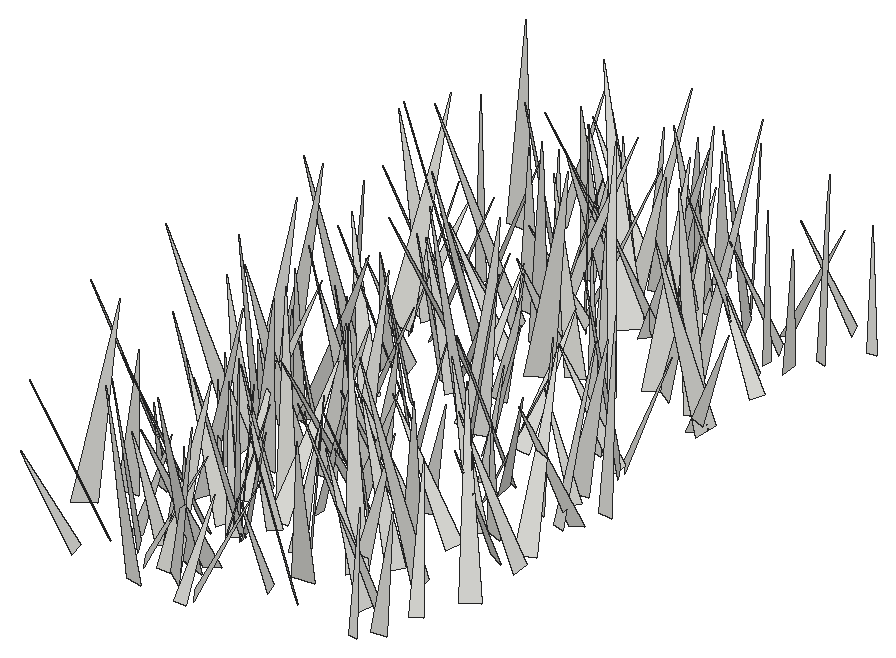
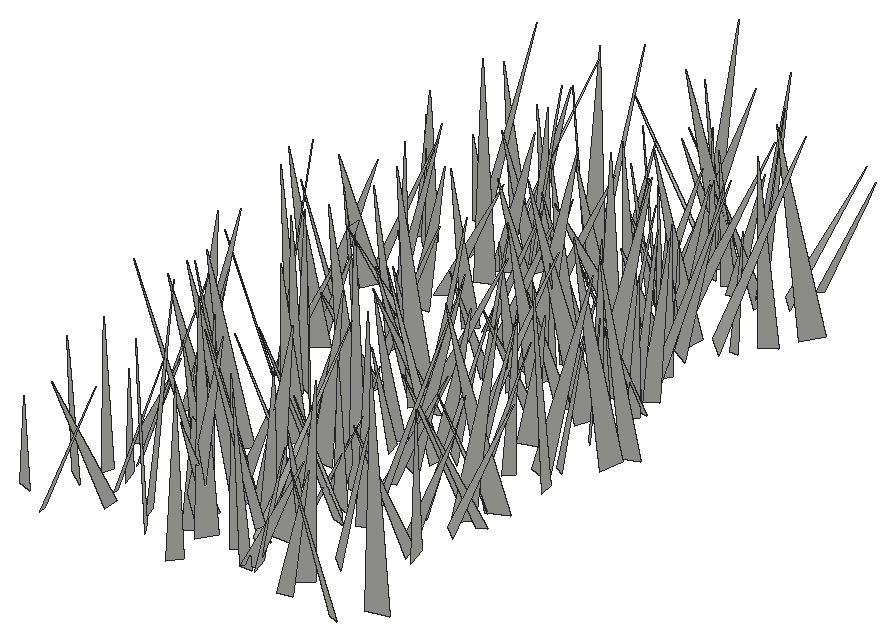
# SketchUp Ruby script. Lengths in inches.
U = 1.inch
M = Sketchup.active_model
def pt(a) = Geom::Point3d.new(a.map { |v| v * U })
def face(e, loops, mat)
  f = e.add_face(loops[0].map { |a| pt(a) })
  loops[1..].each { |l| e.add_face(l.map { |a| pt(a) }).erase! }
  f.material = f.back_material = mat if mat
  f
end
# faces: each face lists its corners as indices into pts; further lists are holes
def faces(e, pts, list, mat = nil) = list.each { |f| face(e, (f[0].is_a?(Array) ? f : [f]).map { |l| l.map { |i| pts[i] } }, mat) }
# xy, xz, yz: faces in a plane at the given z, y or x. An outline is a flat list of corners, or four numbers for a rectangle; further outlines are holes
def ring(l) = l.size == 4 ? [[l[0], l[1]], [l[2], l[1]], [l[2], l[3]], [l[0], l[3]]] : l.each_slice(2).to_a
def flat(e, list, mat, &to3) = list.each { |f| face(e, (f[0].is_a?(Array) ? f : [f]).map { |l| ring(l).map { |u, v| to3.(u, v) } }, mat) }
def xy(e, z, list, mat = nil) = flat(e, list, mat) { |x, y| [x, y, z] }
def xz(e, y, list, mat = nil) = flat(e, list, mat) { |x, z| [x, y, z] }
def yz(e, x, list, mat = nil) = flat(e, list, mat) { |y, z| [x, y, z] }
def lines(e, pts, list) = list.each { |a, b| e.add_line(pt(pts[a]), pt(pts[b])) }
# prism: a flat outline (further loops are holes) pulled along v
def prism(e, loops, v, mat = nil)
  f = face(e, loops, mat); d = Geom::Vector3d.new(v.map { |x| x * U })
  f.pushpull(f.normal.samedirection?(d) ? d.length : -d.length)
end
def box(e, o, s, mat = nil) = prism(e, [[o, [o[0] + s[0], o[1], o[2]], [o[0] + s[0], o[1] + s[1], o[2]], [o[0], o[1] + s[1], o[2]]]], [0, 0, s[2]], mat)
def at(x, y, z, deg = 0) = Geom::Transformation.translation(pt([x, y, z])) * Geom::Transformation.rotation(ORIGIN, Z_AXIS, deg.degrees)
def axes(o, x, y, z) = Geom::Transformation.new([*x, 0, *y, 0, *z, 0, *pt(o).to_a, 1])
def part(name) = M.definitions.add(name)
# library, detail: a bought-in or finely detailed component or shape, given as its bounding box
def library(name, o, s) = part(name).tap { |d| box(d.entities, o, s) }
def detail(e, o, s) = box(e.add_group.entities, o, s)
def put(e, d, t, mat = nil) = e.add_instance(d, t).tap { |i| i.material = mat if mat }
def group(e, t, mat = nil) = e.add_group.tap { |g| g.transformation = t; g.material = mat if mat }.entities
root = M.entities
c1 = part("fur_instance\#9")
p = [[0.8125,0,1.79],[0.67,-0.02,1.48],[0,-0.11,0],[0,0.11,0]]
faces(c1.entities,p,[[0,1,2,3]])
put(root,c1,axes([480.35,103.58,-21.66],[1.05516,-7.50337,2.43147],[-7.87164,-0.84629,0.8044],[0.49989,2.51181,7.53438]))
put(root,c1,axes([480.21,79.61,-21.66],[0.14436,6.2225,2.72909],[6.68972,0.34776,-1.14678],[1.18962,-2.71069,6.11762]))
put(root,c1,axes([483.13,93.17,-21.66],[-3.10953,-4.00727,0.37973],[-3.98696,3.00024,-0.98706],[-0.55366,0.90108,4.97525]))
put(root,c1,axes([480.6,81.01,-21.66],[7.15421,-1.9799,2.12173],[-2.22149,-7.36827,0.61487],[-1.86728,1.18029,7.39761]))
put(root,c1,axes([483.24,84.46,-21.66],[-1.73003,-6.76572,2.01517],[-7.01807,1.42401,-1.24409],[-0.76325,2.2419,6.8717]))
put(root,c1,axes([480.98,61.46,-21.66],[5.12672,-4.5376,2.59386],[-5.0883,-5.16347,1.02416],[-1.19461,2.5199,6.76936]))
put(root,c1,axes([482.8,96.8125,-21.66],[-5.66532,-0.50223,1.85308],[-0.88322,5.80808,-1.12609],[1.70472,1.34012,5.57494]))
put(root,c1,axes([484.51,72.17,-21.66],[-7.8071,-1.03462,1.04066],[-0.93299,7.84786,0.80297],[1.13267,-0.66693,7.83431]))
put(root,c1,axes([483.31,91.69,-21.66],[-5.98098,3.27291,2.42019],[3.72115,6.13978,0.89298],[1.64993,-1.98304,6.75918]))
put(root,c1,axes([484.76,59.01,-21.66],[-3.76268,-4.24685,0.11424],[-4.17448,3.66755,-1.15295],[-0.78896,0.84846,5.55555]))
put(root,c1,axes([482.75,83.29,-21.66],[-2.78076,-3.999,1.01738],[-3.97731,2.92434,0.62365],[1.09912,0.46468,4.83071]))
put(root,c1,axes([484.81,65.8,-21.66],[-4.99858,-6.00178,0.67378],[-6.03784,4.94565,-0.739],[-0.1407,0.9901,7.77567]))
put(root,c1,axes([481.91,85.54,-21.66],[6.17707,1.48648,1.9777],[1.80034,-6.34915,-0.85095],[-1.69697,-1.32504,6.29616]))
put(root,c1,axes([482.12,79.45,-21.66],[3.64013,-0.49009,0.65042],[-0.33955,-3.62113,-0.82821],[-0.74023,-0.74902,3.57838]))
put(root,c1,axes([482.29,89.69,-21.66],[-1.03239,7.59334,1.92082],[7.72051,1.31303,-1.04105],[1.31985,-1.74108,7.59215]))
put(root,c1,axes([484.16,56.68,-21.66],[-3.93279,-0.23592,0.50656],[-0.05149,3.7386,1.34138],[0.55643,-1.32147,3.70448]))
put(root,c1,axes([481.97,91.59,-21.66],[0.26684,4.21608,0.5662],[4.07293,-0.08948,-1.25314],[1.22767,-0.6195,4.03438]))
put(root,c1,axes([482.01,105.68,-21.66],[2.56604,4.25646,1.10853],[4.39439,-2.42581,-0.85772],[0.18887,-1.38883,4.89555]))
put(root,c1,axes([483.74,73.5,-21.66],[3.52477,-3.78027,2.43443],[-3.94318,-4.08529,-0.63451],[-2.1606,1.28874,5.1295]))
put(root,c1,axes([484.54,73.62,-21.66],[-3.5063,-5.04513,2.56803],[-5.65565,3.25438,-1.32851],[0.24851,2.88062,5.99854]))
put(root,c1,axes([482.27,63.98,-21.66],[2.19919,-5.46865,1.19281],[-5.58851,-2.07385,0.79564],[0.31218,1.39943,5.84033]))
put(root,c1,axes([483.25,89.46,-21.66],[3.76197,3.17485,0.58422],[2.97684,-3.75885,1.25811],[-1.24876,0.60394,4.75913]))
put(root,c1,axes([483.43,79.5625,-21.66],[-2.68709,-2.60275,1.28992],[-2.48203,2.97011,0.82256],[1.50922,0.25052,3.6494]))
put(root,c1,axes([484.4,95.37,-21.66],[1.61464,-3.26071,0.69447],[-2.99454,-1.75765,-1.29032],[-1.46534,-0.00102,3.40211]))
put(root,c1,axes([485.8,92.11,-21.66],[-5.67662,-5.13617,1.32256],[-5.29359,5.60645,-0.94818],[0.32758,1.59402,7.59639]))
put(root,c1,axes([483.55,65.67,-21.66],[-0.85908,-3.57953,0.71794],[-3.54097,0.99653,0.73143],[0.88884,0.51028,3.60778]))
put(root,c1,axes([483.27,75.56,-21.66],[4.01305,-1.4697,0.35123],[-1.33059,-3.90931,-1.15533],[-0.71618,-0.97223,4.11458]))
put(root,c1,axes([485.89,100.32,-21.66],[-3.65286,-4.07637,1.60167],[-4.37583,3.48496,-1.11027],[0.18514,1.94004,5.3598]))
put(root,c1,axes([483.44,96.63,-21.66],[4.63443,1.21877,0.59299],[1.09033,-4.6073,0.94811],[-0.80513,0.77609,4.69728]))
put(root,c1,axes([486.17,82.04,-21.66],[-2.8304,4.89567,0.80261],[4.94903,2.72215,0.8485],[-0.34477,-1.11592,5.59096]))
put(root,c1,axes([485.76,68.05,-21.66],[-2.42816,-5.42807,1.43938],[-5.61543,2.33238,-0.67728],[-0.05217,1.5899,5.90772]))
put(root,c1,axes([483.19,74.81,-21.66],[2.79379,4.96818,0.70977],[4.95175,-2.59669,-1.31495],[0.8165,-1.25148,5.54607]))
put(root,c1,axes([484.66,77.3,-21.66],[-1.17903,-5.46423,1.73554],[-5.62366,1.44698,0.7353],[1.11548,1.51937,5.54141]))
put(root,c1,axes([486.03,86.25,-21.66],[-4.24869,-0.73201,1.00331],[-0.4187,4.21079,1.29914],[1.16925,-1.15205,4.11089]))
put(root,c1,axes([484.76,70.5,-21.66],[4.55576,-0.64185,1.19418],[-0.37344,-4.61891,-1.05794],[-1.3033,-0.92017,4.47746]))
put(root,c1,axes([484.73,85.62,-21.66],[4.79188,-1.27621,1.00499],[-1.01396,-4.79557,-1.25507],[-1.26909,-0.98723,4.79746]))
put(root,c1,axes([486.05,105.22,-21.66],[1.60844,-3.68609,1.55705],[-3.78668,-1.94455,-0.69177],[-1.29334,1.10916,3.96179]))
put(root,c1,axes([484.82,89.73,-21.66],[4.77629,1.47467,0.59608],[1.29577,-4.70156,1.24867],[-0.92247,1.03128,4.84029]))
put(root,c1,axes([486.55,74.48,-21.66],[1.44091,-6.85532,1.40735],[-6.89305,-1.6385,-0.92385],[-1.20912,1.1714,6.94393]))
put(root,c1,axes([488.1,93.9,-21.66],[-7.76303,-2.55675,1.09489],[-2.43873,7.81802,0.96517],[1.33728,-0.58482,8.11604]))
put(root,c1,axes([486.87,59.31,-21.66],[-4.89402,-3.33819,1.83703],[-3.30827,5.20635,0.64726],[1.89038,0.46913,5.88863]))
put(root,c1,axes([488.79,63.35,-21.66],[-3.68425,-5.36529,0.32526],[-5.32374,3.58793,-1.11818],[-0.74155,0.8979,6.41168]))
put(root,c1,axes([485.87,60.32,-21.66],[3.36091,-1.13304,0.9234],[-1.35023,-3.29337,0.87337],[-0.55977,1.1411,3.43755]))
put(root,c1,axes([486.125,103.26,-21.66],[4.8862,-3.80667,1.31151],[-3.74132,-5.05482,-0.73291],[-1.48774,0.20937,6.1505]))
put(root,c1,axes([487.35,66.4,-21.66],[-3.69275,-0.52533,1.17947],[-0.76187,3.77166,-0.70545],[1.04243,0.89562,3.66261]))
put(root,c1,axes([486.04,66.42,-21.66],[6.43486,-0.85229,1.84553],[-1.08084,-6.62327,0.70985],[-1.72168,0.97247,6.45212]))
put(root,c1,axes([488.4375,86.17,-21.66],[-2.6227,-3.62693,1.52989],[-3.9333,2.34177,-1.19122],[-0.15598,1.93268,4.31442]))
put(root,c1,axes([487.82,60.39,-21.66],[1.8485,-3.49978,1.33816],[-3.45042,-2.17169,-0.91344],[-1.46071,0.70098,3.8511]))
put(root,c1,axes([488.59,83,-21.66],[-3.38469,-3.26483,1.22467],[-3.48648,3.19729,-1.11215],[0.05857,1.65326,4.56929]))
put(root,c1,axes([489.88,103.8125,-21.66],[-3.98181,3.20015,0.16473],[3.12043,3.81261,1.36007],[-0.7287,-1.16015,4.92402]))
put(root,c1,axes([489.1,64.66,-21.66],[-4.79619,2.23097,0.90337],[2.34699,4.78153,0.65218],[0.53379,-0.97799,5.24932]))
put(root,c1,axes([489.59,90.88,-21.66],[-4.14397,2.00475,0.46664],[2.04964,3.92263,1.34951],[-0.1891,-1.41534,4.40117]))
put(root,c1,axes([488.96,74.16,-21.66],[0.98464,3.25356,1.70885],[3.23357,-1.6077,1.19779],[-1.74639,-1.14237,3.18127]))
put(root,c1,axes([490.18,81.1,-21.66],[-4.77204,-4.71706,0.72174],[-4.75307,4.60775,-1.31181],[-0.42413,1.43592,6.58044]))
put(root,c1,axes([489.4,103.45,-21.66],[-5.02924,-0.94611,0.83871],[-1.10156,4.96734,-1.00192],[0.62059,1.14984,5.01842]))
put(root,c1,axes([485.13,77.6,-21.66],[6.73019,-3.63445,0.24466],[-3.63894,-6.68481,0.79754],[0.16506,0.81773,7.60715]))
put(root,c1,axes([488.13,67.47,-21.66],[-2.89622,3.26829,0.45856],[3.08153,2.89643,-1.18106],[1.18158,0.4572,4.20415]))
put(root,c1,axes([486.59,71.41,-21.66],[1.17018,-6.95871,1.51726],[-7.0392,-0.89595,1.31981],[1.08411,1.69372,6.93189]))
put(root,c1,axes([487.09,77.39,-21.66],[3.48145,-1.92251,0.90917],[-2.10367,-3.36896,0.93158],[-0.31179,1.26381,3.86636]))
put(root,c1,axes([487.35,95.8,-21.66],[0.93072,-6.54849,1.55591],[-6.7031,-0.75944,0.81335],[0.60996,1.64631,6.5641]))
put(root,c1,axes([489.62,88.78,-21.66],[-2.51805,-6.35566,1.6356],[-6.55451,2.34778,-0.96776],[-0.32873,1.87181,6.76746]))
put(root,c1,axes([488.78,69.36,-21.66],[-4.40075,-1.21691,1.44212],[-0.98766,4.60363,0.87078],[1.60783,-0.50284,4.4821]))
put(root,c1,axes([489.28,55.73,-21.66],[1.25077,5.74635,3.18749],[6.40163,-1.79789,0.7292],[-1.48314,-2.91412,5.83551]))
put(root,c1,axes([487.46,101.11,-21.66],[2.40925,-3.29701,1.00546],[-3.44676,-2.29271,0.74099],[0.03277,1.24857,4.01568]))
put(root,c1,axes([487.72,79.45,-21.66],[4.13014,0.16234,0.60229],[0.00137,-4.03539,1.07832],[-0.62379,1.06603,3.99019]))
put(root,c1,axes([489.79,85.53,-21.66],[-3.61147,3.35043,1.62323],[3.67501,3.56996,0.80783],[0.59541,-1.71259,4.85958]))
put(root,c1,axes([489.76,75.13,-21.66],[1.9045,4.44389,1.45881],[4.34306,-2.26488,1.22946],[-1.73613,-0.79091,4.67587]))
put(root,c1,axes([490.43,63.66,-21.66],[-4.5545,1.12209,0.15618],[1.0267,4.36161,-1.39615],[0.47894,1.3207,4.4781]))
put(root,c1,axes([490.03,64.59,-21.66],[-4.76219,-1.42096,1.84075],[-1.91994,4.76946,-1.2853],[1.31199,1.82182,4.80058]))
put(root,c1,axes([490.82,64.08,-21.66],[-2.4507,-4.58404,1.24543],[-4.71435,2.17524,-1.27033],[-0.58261,1.68089,5.0404]))
put(root,c1,axes([490,94.97,-21.66],[1.00537,5.49165,1.69021],[5.63183,-1.28199,0.81538],[-1.13911,-1.49133,5.52306]))
put(root,c1,axes([491.95,85.92,-21.66],[-3.14306,-6.22127,0.26286],[-6.12359,3.03481,-1.39417],[-1.12913,0.859,6.8293]))
put(root,c1,axes([490.93,96.86,-21.66],[-3.84083,-1.16764,0.10273],[-1.10793,3.73134,0.98769],[0.38264,-0.91633,3.89099]))
put(root,c1,axes([491.39,101.33,-21.66],[-5.30348,-5.59312,0.1785],[-5.55783,5.29332,0.73008],[0.65218,-0.37354,7.67313]))
put(root,c1,axes([489.15,95.95,-21.66],[3.76049,3.04894,0.61025],[2.98388,-3.80785,0.6375],[-0.87456,0.11813,4.79905]))
put(root,c1,axes([490.78,68.4,-21.66],[-0.82841,6.75025,1.93378],[7.00258,0.65031,0.72978],[-0.51887,-2.00072,6.76162]))
put(root,c1,axes([488.95,59.54,-21.66],[1.24719,-3.91493,0.4967],[-3.8954,-1.13791,0.81231],[0.63182,0.71228,4.02769]))
put(root,c1,axes([490.55,100.1,-21.66],[1.73584,-5.70606,0.92261],[-5.63591,-1.88469,-1.0526],[-1.28332,0.55882,5.87063]))
put(root,c1,axes([489.92,63.84,-21.66],[3.50829,2.33455,0.59392],[2.17247,-3.51961,1.00185],[-1.04078,0.52272,4.09323]))
put(root,c1,axes([490.28,75.94,-21.66],[-4.55508,3.55475,2.05706],[3.40532,4.98624,-1.07596],[2.29598,-0.34303,5.67691]))
put(root,c1,axes([488.2,58.13,-21.66],[4.34126,2.62004,0.01209],[2.52851,-4.18338,-1.34808],[0.68659,-1.1602,4.88813]))
put(root,c1,axes([489.87,104.11,-21.66],[-1.04898,-5.12431,2.12616],[-5.35306,1.50327,0.98203],[1.45734,1.83333,5.13756]))
put(root,c1,axes([490.1875,59.51,-21.66],[-1.33091,-4.34516,1.37723],[-4.35803,1.6335,0.94222],[1.33595,0.99989,4.44566]))
put(root,c1,axes([493.18,97.96,-21.66],[-5.00695,6.61488,0.9269],[6.67749,4.92855,0.89773],[-0.16413,-1.27989,8.24744]))
put(root,c1,axes([491.8125,60.0625,-21.66],[0.91658,-6.09487,0.23316],[-5.96683,-0.94489,-1.24341],[-1.26442,0.04079,6.03668]))
put(root,c1,axes([491.44,75.21,-21.66],[2.47706,-6.70826,1.39737],[-6.69174,-2.68793,-1.04158],[-1.47445,0.92925,7.07472]))
put(root,c1,axes([489.02,96.39,-21.66],[3.55811,5.92159,0.8478],[5.93377,-3.36884,-1.37307],[0.75783,-1.4247,6.77052]))
put(root,c1,axes([491.61,93.39,-21.66],[1.92833,-3.54748,0.58332],[-3.33012,-2.01195,-1.22706],[-1.35468,-0.10385,3.84674]))
put(root,c1,axes([490.16,57.95,-21.66],[-1.02594,6.32348,2.52203],[6.58274,1.57191,-1.26344],[1.73626,-2.22313,6.28034]))
put(root,c1,axes([491.9375,65.82,-21.66],[1.8151,-3.86013,1.55176],[-3.9232,-2.15155,-0.76319],[-1.38458,1.03602,4.19675]))
put(root,c1,axes([490.86,96.71,-21.66],[5.50119,4.10651,2.99111],[4.73487,-5.74232,-0.82461],[-1.84151,-2.49711,6.81516]))
put(root,c1,axes([490.38,92.84,-21.66],[-1.23371,-7.71978,2.49826],[-7.92295,1.69122,1.31342],[1.75022,2.21429,7.70662]))
put(root,c1,axes([489.07,87.1,-21.66],[6.07626,0.90493,0.17774],[0.92213,-5.94508,-1.25588],[0.01299,-1.26833,6.01354]))
put(root,c1,axes([490.71,64.0625,-21.66],[4.61711,2.95667,1.94744],[3.35791,-4.67134,-0.86895],[-1.12198,-1.8135,5.41336]))
put(root,c1,axes([492.35,98.92,-21.66],[-0.54447,5.56352,1.73211],[5.79599,0.33809,0.73596],[-0.59958,-1.78391,5.54144]))
put(root,c1,axes([490.27,72.75,-21.66],[2.54415,-5.74451,1.38415],[-5.89364,-2.3587,1.04378],[0.42454,1.68081,6.19537]))
put(root,c1,axes([490.88,59.28,-21.66],[-1.24529,-7.71146,0.7872],[-7.61167,1.36728,1.35282],[1.46589,0.54863,7.69333]))
put(root,c1,axes([491.42,66.81,-21.66],[-1.51981,5.35977,0.02073],[5.22969,1.48762,-1.21441],[1.17387,0.31183,5.43711]))
put(root,c1,axes([490.78,77.55,-21.66],[2.11868,-4.0714,0.72457],[-4.11944,-2.00647,0.77101],[0.3627,0.99394,4.52445]))
put(root,c1,axes([490.96,57.56,-21.66],[-2.2184,-4.85625,2.50772],[-5.03427,2.86928,1.10295],[2.1279,1.72546,5.22379]))
put(root,c1,axes([493.1,77.57,-21.66],[-3.89447,-3.70378,1.65585],[-4.00703,3.87088,-0.766],[0.63525,1.71028,5.3196]))
put(root,c1,axes([492.05,87.43,-21.66],[3.63401,0.67625,1.41653],[0.37628,-3.84346,0.86953],[-1.5239,0.6636,3.59267]))
put(root,c1,axes([490.95,64.27,-21.66],[4.30698,0.82715,0.77594],[0.97071,-4.26434,-0.84231],[-0.5865,-0.98365,4.30404]))
put(root,c1,axes([494.1,81.43,-21.66],[-7.25051,-1.24633,1.39987],[-1.43303,7.2913,-0.93068],[1.20805,1.16894,7.29774]))
put(root,c1,axes([491.34,100.63,-21.66],[2.79902,6.82497,1.56007],[7.00009,-2.70115,-0.74237],[0.11309,-1.72399,7.33919]))
put(root,c1,axes([494.2,71.48,-21.66],[-1.56968,-5.60909,0.11931],[-5.50885,1.51747,-1.1357],[-1.06238,0.41882,5.71278]))
put(root,c1,axes([490.32,97.42,-21.66],[5.45999,3.37552,0.2587],[3.37248,-5.38033,-0.97518],[0.29572,-0.96459,6.34466]))
put(root,c1,axes([491.66,102.5625,-21.66],[2.32363,-4.81619,0.47979],[-4.81966,-2.25368,0.71896],[0.44354,0.74187,5.29887]))
put(root,c1,axes([494.3125,91.39,-21.66],[-1.23354,6.12021,2.2306],[6.48252,0.93032,1.03231],[-0.63996,-2.37312,6.15735]))
put(root,c1,axes([492.67,69.15,-21.66],[4.75143,0.92242,1.33841],[0.70934,-4.89704,0.85681],[-1.46255,0.62163,4.7637]))
put(root,c1,axes([492.85,82.59,-21.66],[-0.26942,5.43204,0.24352],[5.36362,0.30555,-0.88154],[0.89325,-0.19629,5.36679]))
put(root,c1,axes([493.05,55.42,-21.66],[-0.85161,3.55792,0.87868],[3.50079,1.05663,-0.88551],[1.08413,-0.61714,3.54963]))
put(root,c1,axes([492.45,86.52,-21.66],[1.94389,-4.04886,0.80465],[-4.08173,-1.75236,1.04312],[0.61659,1.16421,4.36851]))
put(root,c1,axes([493.51,76.89,-21.66],[3.85077,0.95797,1.10657],[0.6489,-3.90916,1.12606],[-1.31192,0.87829,3.80501]))
put(root,c1,axes([492.52,90.21,-21.66],[5.49312,-5.94068,1.74056],[-6.16398,-5.4638,0.80479],[-0.57141,1.8305,8.05098]))
put(root,c1,axes([495.29,73.25,-21.66],[-1.01525,-4.25558,0.24661],[-4.20456,0.95799,-0.77812],[-0.70176,0.41691,4.30525]))
put(root,c1,axes([494.67,71.22,-21.66],[-2.5051,-3.46967,0.23869],[-3.39401,2.50314,0.76559],[0.75915,-0.25846,4.21047]))
put(root,c1,axes([495.52,98.03,-21.66],[-0.21744,-4.53269,0.61909],[-4.46943,0.07824,-0.99696],[-0.9761,0.65149,4.42703]))
put(root,c1,axes([493.79,105.98,-21.66],[4.8037,-2.51399,0.9877],[-2.43404,-4.90267,-0.64073],[-1.17095,-0.12226,5.38379]))
put(root,c1,axes([495.56,102.32,-21.66],[0.0044,-6.27087,2.13822],[-6.5778,-0.25997,-0.7489],[-0.79272,2.12236,6.226]))
put(root,c1,axes([493.87,82.38,-21.66],[-3.12669,6.25889,3.83958],[6.87271,3.96367,-0.86451],[2.58493,-2.9678,6.9428]))
put(root,c1,axes([494.65,64.58,-21.66],[3.28542,-2.52777,1.83261],[-2.97263,-3.34603,0.71392],[-0.95477,1.71946,4.08337]))
put(root,c1,axes([496.68,72.64,-21.66],[-4.54566,0.43172,0.55069],[0.54174,4.46219,0.97364],[0.44289,-1.02717,4.4611]))
put(root,c1,axes([495.37,100.43,-21.66],[-3.3116,2.69695,0.72945],[2.42136,3.33487,-1.33716],[1.39378,0.61437,4.05614]))
put(root,c1,axes([495.05,80.22,-21.66],[4.98467,2.72403,1.68688],[2.57744,-5.26236,0.88159],[-1.90334,0.00786,5.61161]))
put(root,c1,axes([493.16,56.64,-21.66],[4.26257,2.91433,0.00484],[2.86478,-4.18851,-0.95515],[0.53516,-0.79116,5.0745]))
put(root,c1,axes([496.79,68.91,-21.66],[-6.4254,-4.61842,2.37343],[-5.01235,6.50279,-0.91585],[1.35622,2.15235,7.85982]))
put(root,c1,axes([494.05,102.625,-21.66],[6.83248,-2.68093,1.04491],[-2.55055,-6.88917,-0.99801],[-1.33189,-0.56029,7.27146]))
put(root,c1,axes([493.86,71.21,-21.66],[3.98681,-3.04122,0.56389],[-3.08769,-3.85909,1.01744],[0.18196,1.14894,4.91004]))
put(root,c1,axes([496.16,60.16,-21.66],[-3.36385,-0.86607,1.07357],[-0.51946,3.41676,1.12873],[1.27781,-0.89095,3.28504]))
put(root,c1,axes([497.1,90.52,-21.66],[5.53383,-2.65462,5.00816],[-4.23304,-6.59023,1.18414],[-3.76962,3.5034,6.0223]))
put(root,c1,axes([495.93,80.93,-21.66],[4.26152,0.65659,1.09682],[0.47447,-4.35714,0.76482],[-1.18701,0.6156,4.24343]))
put(root,c1,axes([495.22,102.52,-21.66],[5.27759,-3.33069,0.22963],[-3.2336,-5.20637,-1.19863],[-0.83073,-0.89406,6.12452]))
put(root,c1,axes([495.87,64.26,-21.66],[4.89735,3.35239,2.18214],[3.80193,-4.97328,-0.89225],[-1.24321,-2.00306,5.86741]))
put(root,c1,axes([497.68,98.25,-21.66],[0.68594,6.83231,0.78357],[6.74689,-0.82108,1.2531],[-1.33188,-0.64057,6.75135]))
put(root,c1,axes([499.02,64.83,-21.66],[-7.08431,2.74004,0.68893],[2.60293,7.0529,-1.28499],[1.09872,0.95845,7.48626]))
put(root,c1,axes([494.73,98.1,-21.66],[7.07738,-3.29601,0.99897],[-3.4049,-7.03943,0.89669],[-0.51794,1.23844,7.75557]))
put(root,c1,axes([496.49,99.85,-21.66],[1.50872,-5.62418,0.24688],[-5.60162,-1.47433,0.64555],[0.56049,0.40439,5.78713]))
put(root,c1,axes([497.95,60.29,-21.66],[-3.94207,-4.94022,1.13908],[-4.81769,4.09962,1.10733],[1.57897,0.1748,6.2225]))
put(root,c1,axes([497.36,82.43,-21.66],[-1.55041,4.4226,0.08121],[4.26043,1.51619,-1.23272],[1.18941,0.33394,4.52145]))
put(root,c1,axes([499.59,78.96,-21.66],[-3.22494,-3.97651,0.65226],[-4.0077,3.07801,-1.05003],[-0.42001,1.16258,5.01102]))
put(root,c1,axes([497.95,78.11,-21.66],[-3.37958,0.77927,1.41196],[0.41341,3.58754,-0.99047],[1.55884,0.73803,3.32382]))
put(root,c1,axes([497.5,104.12,-21.66],[5.0794,2.90769,2.21904],[3.29641,-5.28463,-0.62087],[-1.58507,-1.67247,5.81975]))
put(root,c1,axes([497.01,62.19,-21.66],[1.92624,-6.27783,0.49509],[-6.26935,-1.863,0.76884],[0.59288,0.69623,6.52153]))
put(root,c1,axes([498.56,102.49,-21.66],[-6.30807,-3.21691,2.7037],[-2.95993,6.86307,1.25992],[2.98285,0.00727,6.96799]))
put(root,c1,axes([500.51,66.61,-21.66],[-3.89894,3.87426,1.21258],[4.05705,3.77806,0.97396],[0.14352,-1.54866,5.40953]))
put(root,c1,axes([497.64,73.09,-21.66],[2.67886,-4.09104,0.57639],[-4.11516,-2.58128,0.80469],[0.36641,0.91951,4.82342]))
put(root,c1,axes([499.08,93.07,-21.66],[-4.71435,5.59524,2.23508],[5.56124,5.13291,-1.11952],[2.31839,-0.93486,7.23039]))
put(root,c1,axes([501.49,70.97,-21.66],[-4.58774,2.19144,0.09862],[2.15217,4.45217,1.18567],[-0.42461,-1.11142,4.94408]))
put(root,c1,axes([498.74,65.45,-21.66],[4.04203,-2.33275,1.48439],[-2.65208,-4.01454,0.91276],[-0.78205,1.55722,4.57675]))
put(root,c1,axes([501.54,73.14,-21.66],[-2.10663,5.00928,1.58804],[5.23429,1.84857,1.1125],[-0.46582,-1.88217,5.31913]))
put(root,c1,axes([500.87,85.01,-21.66],[1.52535,6.05061,2.3847],[6.37233,-1.8801,0.69429],[-1.30004,-2.1163,6.20117]))
put(root,c1,axes([503.08,61.97,-21.66],[-6.30191,-3.29477,0.26908],[-3.30318,6.25333,-0.79169],[-0.13009,0.82599,7.06702]))
put(root,c1,axes([501.28,85.14,-21.66],[1.52535,6.57132,1.88983],[6.63248,-1.89273,1.22809],[-1.66251,-1.52175,6.63331]))
put(root,c1,axes([499.88,96.12,-21.66],[3.85814,7.37241,1.12129],[7.37277,-3.96052,0.67189],[-1.11889,-0.67587,8.29374]))
put(root,c1,axes([499.5,76.18,-21.66],[4.18382,1.92252,0.07247],[1.86113,-4.08842,1.01327],[-0.48737,0.89131,4.49152]))
put(root,c1,axes([502.11,61.82,-21.66],[-4.9541,1.83691,1.27432],[2.05779,4.95762,0.85363],[0.87385,-1.26054,5.21428]))
put(root,c1,axes([501.75,101.67,-21.66],[-4.09527,-2.1175,0.66115],[-1.87882,4.04889,1.32991],[1.17939,-0.90267,4.41434]))
put(root,c1,axes([499.85,93,-21.66],[3.01267,4.99828,1.819],[5.31773,-2.78497,-1.15474],[0.11548,-2.15148,5.72063]))
put(root,c1,axes([502.13,99.87,-21.66],[-4.48133,-0.60292,1.35721],[-0.97091,4.45413,-1.22715],[1.12377,1.44397,4.35201]))
put(root,c1,axes([502.91,97.95,-21.66],[-6.09562,-2.74651,0.83103],[-2.67616,6.14538,0.68045],[1.03541,-0.28555,6.65108]))
put(root,c1,axes([499.62,78,-21.66],[4.97063,-0.22915,0.23226],[-0.15729,-4.7897,-1.3593],[-0.28585,-1.34904,4.78665]))
put(root,c1,axes([503.07,65.84,-21.66],[-7.82049,-1.65264,1.82204],[-1.48703,8.01344,0.88582],[1.95953,-0.51451,7.94397]))
put(root,c1,axes([503.34,84.32,-21.66],[-4.40105,0.97982,0.44244],[1.06612,4.21791,1.26401],[0.13855,-1.33202,4.328]))
put(root,c1,axes([500.36,68.3,-21.66],[1.17808,-6.7396,1.1437],[-6.76699,-0.98532,1.16408],[0.96855,1.31342,6.74203]))
put(root,c1,axes([502.85,92.28,-21.66],[1.15068,-6.84996,3.27998],[-7.48842,-1.57649,-0.66528],[-1.26644,3.09791,6.914]))
put(root,c1,axes([504.24,96.33,-21.66],[-3.16167,2.60611,0.16715],[2.5519,3.02748,1.0668],[-0.55458,-0.92652,3.956]))
put(root,c1,axes([503.9,79.45,-21.66],[-1.40668,3.30295,0.84871],[3.29754,1.08331,1.24951],[-0.86952,-1.23511,3.36556]))
put(root,c1,axes([502.96,77.33,-21.66],[2.73063,4.59292,1.67983],[4.59916,-3.06583,0.90635],[-1.66266,-0.93747,5.2659]))
put(root,c1,axes([500.97,103.13,-21.66],[4.26787,-0.90452,0.30078],[-0.95208,-4.11231,1.14272],[-0.04649,1.18073,4.21035]))
put(root,c1,axes([504.12,91.62,-21.66],[-4.01169,-3.78695,1.3287],[-4.00574,3.89344,-0.9976],[0.2459,1.64323,5.42581]))
put(root,c1,axes([503.71,106.17,-21.66],[-4.07009,-1.55263,0.42821],[-1.43545,4.0247,0.94922],[0.73043,-0.7422,4.25151]))
put(root,c1,axes([503.59,58.68,-21.66],[0.89714,3.83975,1.01573],[3.88067,-1.06922,0.61438],[-0.84607,-0.83267,3.89501]))
put(root,c1,axes([503.45,84.2,-21.66],[-6.01698,-4.0059,2.23214],[-3.85326,6.41302,1.12219],[2.48637,0.24439,7.14087]))
put(root,c1,axes([502.48,73.43,-21.66],[-0.50328,-4.91347,1.0032],[-4.85841,0.72759,1.12622],[1.24277,0.85458,4.80907]))
put(root,c1,axes([504.47,91.125,-21.66],[-6.49711,1.14641,2.18071],[1.63194,6.61021,1.38712],[1.84567,-1.80917,6.45001]))
put(root,c1,axes([504.61,101.9,-21.66],[2.34142,5.16985,1.64131],[5.10687,-2.70355,1.23051],[-1.82787,-0.93109,5.54034]))
put(root,c1,axes([505.07,62.86,-21.66],[-0.56854,4.75375,0.07359],[4.64609,0.5398,1.02436],[-1.0087,-0.19303,4.67676]))
put(root,c1,axes([504.36,71.31,-21.66],[-1.82022,-4.66244,0.24993],[-4.60062,1.83672,0.75812],[0.79693,-0.04591,4.9474]))
put(root,c1,axes([503.64,100.0625,-21.66],[4.65785,-0.69082,1.21899],[-0.53967,-4.78978,-0.65231],[-1.29303,-0.48941,4.6634]))
put(root,c1,axes([506.3,71.25,-21.66],[-5.398,0.07669,0.31538],[0.11355,5.36878,0.63804],[0.30406,-0.64352,5.36071]))
put(root,c1,axes([505.45,72.72,-21.66],[-4.47188,4.60163,0.40246],[4.4512,4.44255,-1.33612],[1.23441,0.65071,6.27595]))
put(root,c1,axes([504.88,76.62,-21.66],[2.36342,5.34352,0.74133],[5.25737,-2.46286,0.99138],[-1.20944,-0.26392,5.75813]))
put(root,c1,axes([503.2,80.5,-21.66],[2.93008,-5.46925,1.49234],[-5.65269,-2.69042,1.23848],[0.43226,1.89052,6.07982]))
put(root,c1,axes([505.62,77.45,-21.66],[0.74185,-5.118,0.35857],[-5.01336,-0.80012,-1.04825],[-1.09027,0.19676,5.06413]))
put(root,c1,axes([506.5,66.23,-21.66],[-2.09458,6.39775,0.76013],[6.40195,1.97698,1.00139],[-0.72385,-1.02792,6.657]))
put(root,c1,axes([503.4,84.73,-21.66],[3.56732,3.05528,0.6125],[3.0981,-3.37772,-1.19517],[0.33415,-1.30074,4.54225]))
put(root,c1,axes([506.01,67.11,-21.66],[2.91004,3.86675,2.0314],[3.84438,-3.42612,1.0144],[-2.0734,-0.92551,4.73192]))
put(root,c1,axes([504.6,59.91,-21.66],[1.60896,-4.17155,1.4473],[-4.41412,-1.4813,0.63763],[0.1098,1.57772,4.42538]))
put(root,c1,axes([503.92,90.64,-21.66],[3.45367,-2.54495,0.42724],[-2.57712,-3.36456,0.79082],[0.1334,0.88889,4.21654]))
put(root,c1,axes([506.25,104.66,-21.66],[0.5097,3.85536,0.87755],[3.83119,-0.70034,0.85159],[-0.9777,-0.73445,3.79452]))
put(root,c1,axes([506.15,79.48,-21.66],[1.54209,5.92638,1.72605],[6.04197,-1.81335,0.82809],[-1.2633,-1.43843,6.06748]))
